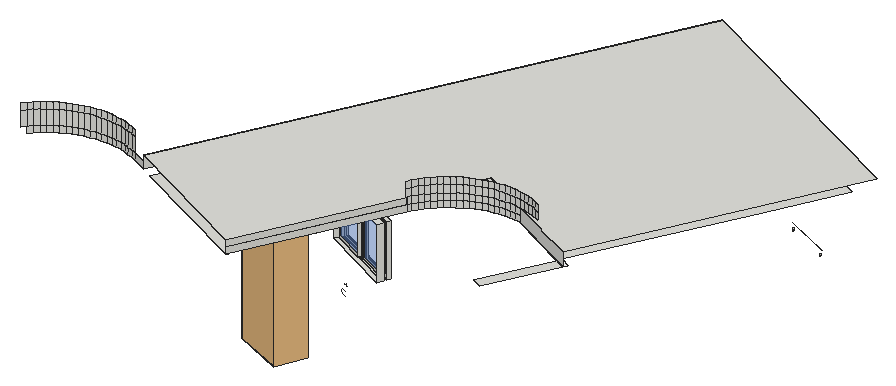
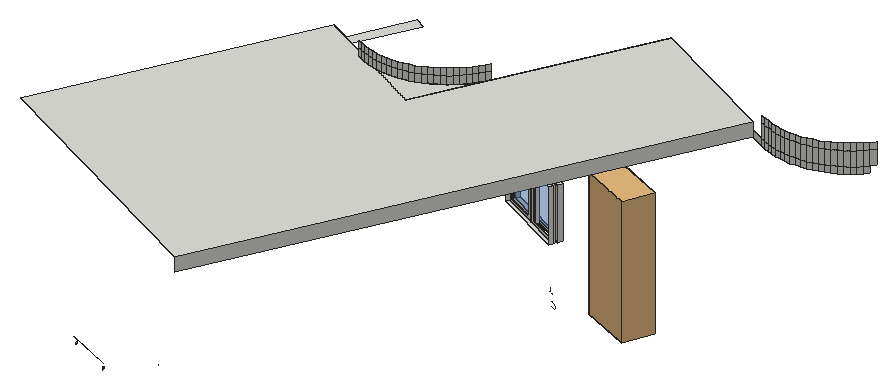
# SketchUp Ruby script. Lengths in inches.
U = 1.inch
M = Sketchup.active_model
def pt(a) = Geom::Point3d.new(a.map { |v| v * U })
def face(e, loops, mat)
  f = e.add_face(loops[0].map { |a| pt(a) })
  loops[1..].each { |l| e.add_face(l.map { |a| pt(a) }).erase! }
  f.material = f.back_material = mat if mat
  f
end
# faces: each face lists its corners as indices into pts; further lists are holes
def faces(e, pts, list, mat = nil) = list.each { |f| face(e, (f[0].is_a?(Array) ? f : [f]).map { |l| l.map { |i| pts[i] } }, mat) }
# xy, xz, yz: faces in a plane at the given z, y or x. An outline is a flat list of corners, or four numbers for a rectangle; further outlines are holes
def ring(l) = l.size == 4 ? [[l[0], l[1]], [l[2], l[1]], [l[2], l[3]], [l[0], l[3]]] : l.each_slice(2).to_a
def flat(e, list, mat, &to3) = list.each { |f| face(e, (f[0].is_a?(Array) ? f : [f]).map { |l| ring(l).map { |u, v| to3.(u, v) } }, mat) }
def xy(e, z, list, mat = nil) = flat(e, list, mat) { |x, y| [x, y, z] }
def xz(e, y, list, mat = nil) = flat(e, list, mat) { |x, z| [x, y, z] }
def yz(e, x, list, mat = nil) = flat(e, list, mat) { |y, z| [x, y, z] }
def lines(e, pts, list) = list.each { |a, b| e.add_line(pt(pts[a]), pt(pts[b])) }
# prism: a flat outline (further loops are holes) pulled along v
def prism(e, loops, v, mat = nil)
  f = face(e, loops, mat); d = Geom::Vector3d.new(v.map { |x| x * U })
  f.pushpull(f.normal.samedirection?(d) ? d.length : -d.length)
end
def box(e, o, s, mat = nil) = prism(e, [[o, [o[0] + s[0], o[1], o[2]], [o[0] + s[0], o[1] + s[1], o[2]], [o[0], o[1] + s[1], o[2]]]], [0, 0, s[2]], mat)
def at(x, y, z, deg = 0) = Geom::Transformation.translation(pt([x, y, z])) * Geom::Transformation.rotation(ORIGIN, Z_AXIS, deg.degrees)
def axes(o, x, y, z) = Geom::Transformation.new([*x, 0, *y, 0, *z, 0, *pt(o).to_a, 1])
def part(name) = M.definitions.add(name)
# library, detail: a bought-in or finely detailed component or shape, given as its bounding box
def library(name, o, s) = part(name).tap { |d| box(d.entities, o, s) }
def detail(e, o, s) = box(e.add_group.entities, o, s)
def put(e, d, t, mat = nil) = e.add_instance(d, t).tap { |i| i.material = mat if mat }
def group(e, t, mat = nil) = e.add_group.tap { |g| g.transformation = t; g.material = mat if mat }.entities
root = M.entities
M.materials.add("Glass_Safety_01").color = [204, 235, 244]
M.materials["Glass_Safety_01"].alpha = 0.1
M.materials.add("[Color_000]").color = [255, 255, 255]
M.materials.add("[Translucent Glass Blue]").color = [100, 149, 237]
M.materials["[Translucent Glass Blue]"].alpha = 0.5
c1 = library("Shower_03.skp",[-9.2,-8.46,-0.03],[13.92,58.47,24.25])
c2 = part("Janela aluminio")
xy(c2.entities,0,[[0,0,47.24,1.57],[23.62,1.57,47.24,2.76],[0,2.76,25.98,3.9375],[0,3.9375,47.24,5.91]])
xy(c2.entities,43.31,[[0,0,47.24,1.57],[23.62,1.57,47.24,2.76],[0,2.76,0,5.91,47.24,5.91,47.24,3.9375,25.98,3.9375,25.98,2.76],[25.98,2.76,47.24,3.9375]])
xz(c2.entities,1.57,[[0,0,23.62,0,23.62,41.34,21.26,41.34,21.26,1.97,1.97,1.97,1.97,41.34,23.62,41.34,23.62,43.31,0,43.31],[[23.62,0,47.24,43.31],[25.7,1.97,45.28,41.34]]])
xz(c2.entities,2.76,[[[0,0,23.62,43.31],[2.36,2.36,21.26,40.94]],[23.62,0,25.98,43.31]])
xz(c2.entities,2.76,[[2.36,2.36,21.26,40.94]],"[Translucent Glass Blue]")
xz(c2.entities,3.9375,[[25.98,0,25.98,2.36,44.88,2.36,44.88,40.94,25.98,40.94,25.98,43.31,47.24,43.31,47.24,0]])
xz(c2.entities,3.9375,[[25.98,2.36,44.88,40.94]],"[Translucent Glass Blue]")
yz(c2.entities,0,[[0,0,1.57,43.31],[2.76,0,5.91,43.31]])
yz(c2.entities,23.62,[[1.57,0,2.76,43.31]])
yz(c2.entities,25.98,[[2.76,0,3.9375,43.31]])
yz(c2.entities,47.24,[[0,0,1.57,43.31],[1.57,0,2.76,43.31],[3.9375,0,5.91,43.31]])
xy(root,354.51,[[846.73,1089.54,846.8,1089.72,825.62,1098.73],[846.8,1089.72,825.7,1098.91,825.62,1098.73]],"Glass_Safety_01")
xy(root,412.84,[[744.84,871.72,744.58,871.85,776.25,937.08,776.52,936.95],[744.57,871.86,686.94,899.84,784.83,1101.43,892.64,1049.08,877.08,1017.03,841.92,944.62,824.11,953.26,821.96,954.22,819.75,955.04,817.49,955.71,815.2,956.23,812.87,956.6,790.91,967.26,776.25,937.08,776,936.6],[831.12,910.93,845.58,940.71,841.08,942.9,826.625,913.12],[776.25,937.08,790.91,967.26,812.87,956.6,810.52,956.81,808.17,956.88,805.8125,956.79,803.47,956.54,801.15,956.14,798.86,955.59,796.61,954.9,794.41,954.05,792.27,953.07,790.2,951.94,788.21,950.6875,786.3,949.3,784.49,947.8,782.78,946.18,781.18,944.45,779.69,942.62,778.33,940.7,777.1,938.6875],[841.08,942.9,812.87,956.6,815.2,956.23,817.49,955.71,819.75,955.04,821.96,954.22,824.11,953.26,841.92,944.62]])
xy(root,412.84,[[845.58,940.71,846.42,942.43,841.92,944.62,841.08,942.9]],"[Color_000]")
xy(root,415.76,[[744.84,871.72,744.57,871.86,776,936.6,776.25,937.08,776.52,936.95]])
xy(root,418.84,[[744.57,871.86,776,936.6,776.25,937.08,790.91,967.26,812.87,956.6,845.58,940.71,900.47,1053.75,783.66,1110.47,682.44,902.02],[776.25,937.08,777.1,938.6875,778.33,940.7,779.69,942.62,781.18,944.45,782.78,946.18,784.49,947.8,786.3,949.3,788.21,950.6875,790.2,951.94,792.27,953.07,794.41,954.05,796.61,954.9,798.86,955.59,801.15,956.14,803.47,956.54,805.8125,956.79,808.17,956.88,810.52,956.81,812.87,956.6,790.91,967.26]])
p = [[845.78,1089.95,352.07],[845.88,1089.9,351.8125],[845.77,1089.65,351.8125],[845.67,1089.69,352.07],[826.59,1098.3,351.8125],[826.69,1098.26,352.07],
  [826.58,1098.01,352.07],[826.48,1098.05,351.8125],[845.75,1089.96,352.35],[845.64,1089.71,352.35],[826.73,1098.25,352.35],[826.62,1097.99,352.35],
  [845.78,1089.95,352.62],[845.67,1089.69,352.62],[826.69,1098.26,352.62],[826.58,1098.01,352.62],[826.59,1098.3,352.88],[826.48,1098.05,352.88],
  [744.84,871.72,412.84],[776.52,936.95,412.84],[776.52,936.95,415.76],[744.84,871.72,415.76],[776,936.6,412.84],[744.57,871.86,412.84],
  [744.57,871.86,415.76],[776,936.6,415.76],[634.24,898.27,415.76],[634.24,898.27,412.84],[632.64,896.54,412.84],[632.64,896.54,415.76],
  [635.95,899.89,415.76],[635.95,899.89,412.84],[637.76,901.4,415.76],[637.76,901.4,412.84],[639.67,902.78,415.76],[639.67,902.78,412.84],
  [675.58,905.36,415.76],[682.44,902.02,415.76],[682.44,902.02,412.84],[675.58,905.36,412.84],[780.62,1104.21,412.84],[682.44,902.02,418.84],
  [783.66,1110.47,418.84],[783.66,1110.47,412.84],[641.66,904.04,415.76],[641.66,904.04,412.84],[643.73,905.16,415.76],[643.73,905.16,412.84],
  [645.875,906.15,415.76],[645.875,906.15,412.84],[673.43,906.3125,412.84],[673.43,906.3125,415.76],[648.07,906.99,415.76],[648.07,906.99,412.84],
  [671.22,907.13,412.84],[671.22,907.13,415.76],[650.32,907.6875,415.76],[650.32,907.6875,412.84],[668.96,907.8,412.84],[668.96,907.8,415.76],
  [652.61,908.24,415.76],[652.61,908.24,412.84],[666.66,908.32,412.84],[666.66,908.32,415.76],[654.9375,908.63,415.76],[654.9375,908.63,412.84],
  [664.33,908.69,412.84],[664.33,908.69,415.76],[657.28,908.88,415.76],[657.28,908.88,412.84],[661.99,908.91,412.84],[661.99,908.91,415.76],
  [659.63,908.97,415.76],[659.63,908.97,412.84],[776.25,937.08,415.76],[776.25,937.08,412.84],[777.1,938.6875,412.84],[777.1,938.6875,415.76],
  [790.91,967.26,412.84],[790.91,967.26,418.84],[776.25,937.08,418.84],[778.33,940.7,412.84],[778.33,940.7,415.76],[779.69,942.62,412.84],
  [779.69,942.62,415.76],[845.58,940.71,418.84],[812.87,956.6,418.84],[812.87,956.6,415.76],[812.87,956.6,412.84],[841.08,942.9,412.84],
  [845.58,940.71,412.84],[781.18,944.45,412.84],[781.18,944.45,415.76],[782.78,946.18,412.84],[782.78,946.18,415.76],[784.49,947.8,412.84],
  [784.49,947.8,415.76],[786.3,949.3,412.84],[786.3,949.3,415.76],[788.21,950.6875,412.84],[788.21,950.6875,415.76],[790.2,951.94,412.84],
  [790.2,951.94,415.76],[792.27,953.07,412.84],[792.27,953.07,415.76],[794.41,954.05,412.84],[794.41,954.05,415.76],[824.11,953.26,415.76],
  [824.11,953.26,412.84],[821.96,954.22,412.84],[821.96,954.22,415.76],[796.61,954.9,412.84],[796.61,954.9,415.76],[819.75,955.04,412.84],
  [819.75,955.04,415.76],[798.86,955.59,412.84],[798.86,955.59,415.76],[817.49,955.71,412.84],[817.49,955.71,415.76],[801.15,956.14,412.84],
  [801.15,956.14,415.76],[815.2,956.23,412.84],[815.2,956.23,415.76],[803.47,956.54,412.84],[803.47,956.54,415.76],[805.8125,956.79,412.84],
  [805.8125,956.79,415.76],[810.52,956.81,415.76],[810.52,956.81,412.84],[808.17,956.88,412.84],[808.17,956.88,415.76],[776,936.6,418.84],
  [744.57,871.86,418.84],[631.16,894.71,415.76],[631.16,894.71,422.51],[632.64,896.54,422.51],[634.24,898.27,422.51],[635.95,899.89,422.51],
  [637.76,901.4,422.51],[639.67,902.78,422.51],[641.66,904.04,422.51],[643.73,905.16,422.51],[645.875,906.15,422.51],[673.43,906.3125,422.51],
  [675.58,905.36,422.51],[648.07,906.99,422.51],[671.22,907.13,422.51],[650.32,907.6875,422.51],[668.96,907.8,422.51],[652.61,908.24,422.51],
  [666.66,908.32,422.51],[654.9375,908.63,422.51],[664.33,908.69,422.51],[657.28,908.88,422.51],[661.99,908.91,422.51],[659.63,908.97,422.51],
  [777.1,938.6875,418.84],[778.33,940.7,418.84],[779.69,942.62,418.84],[781.18,944.45,418.84],[782.78,946.18,418.84],[784.49,947.8,418.84],
  [786.3,949.3,418.84],[788.21,950.6875,418.84],[790.2,951.94,418.84],[792.27,953.07,418.84],[794.41,954.05,418.84],[821.96,954.22,422.51],
  [824.11,953.26,422.51],[796.61,954.9,418.84],[819.75,955.04,422.51],[798.86,955.59,418.84],[817.49,955.71,422.51],[801.15,956.14,418.84],
  [815.2,956.23,422.51],[803.47,956.54,418.84],[812.87,956.6,422.51],[805.8125,956.79,418.84],[810.52,956.81,418.84],[808.17,956.88,418.84],
  [777.1,938.6875,422.51],[776,936.6,422.51],[778.33,940.7,422.51],[779.69,942.62,422.51],[781.18,944.45,422.51],[782.78,946.18,422.51],
  [784.49,947.8,422.51],[786.3,949.3,422.51],[788.21,950.6875,422.51],[790.2,951.94,422.51],[792.27,953.07,422.51],[794.41,954.05,422.51],
  [796.61,954.9,422.51],[798.86,955.59,422.51],[801.15,956.14,422.51],[803.47,956.54,422.51],[805.8125,956.79,422.51],[810.52,956.81,422.51],
  [808.17,956.88,422.51],[631.16,894.71,425.53],[632.64,896.54,425.53],[634.24,898.27,425.53],[635.95,899.89,425.53],[637.76,901.4,425.53],
  [639.67,902.78,425.53],[641.66,904.04,425.53],[643.73,905.16,425.53],[645.875,906.15,425.53],[673.43,906.3125,425.53],[675.58,905.36,425.53],
  [648.07,906.99,425.53],[671.22,907.13,425.53],[650.32,907.6875,425.53],[668.96,907.8,425.53],[652.61,908.24,425.53],[666.66,908.32,425.53],
  [654.9375,908.63,425.53],[664.33,908.69,425.53],[657.28,908.88,425.53],[661.99,908.91,425.53],[659.63,908.97,425.53],[776,936.6,425.53],
  [777.1,938.6875,425.53],[778.33,940.7,425.53],[779.69,942.62,425.53],[781.18,944.45,425.53],[782.78,946.18,425.53],[784.49,947.8,425.53],
  [786.3,949.3,425.53],[788.21,950.6875,425.53],[790.2,951.94,425.53],[792.27,953.07,425.53],[794.41,954.05,425.53],[821.96,954.22,425.53],
  [824.11,953.26,425.53],[796.61,954.9,425.53],[819.75,955.04,425.53],[798.86,955.59,425.53],[817.49,955.71,425.53],[801.15,956.14,425.53],
  [815.2,956.23,425.53],[803.47,956.54,425.53],[812.87,956.6,425.53],[805.8125,956.79,425.53],[810.52,956.81,425.53],[808.17,956.88,425.53],
  [729.23,959.8,356.46],[729.1875,959.88,356.41],[729.16,959.95,356.4],[729.34,959.68,356.5],[729.48,959.59,356.52],[729.63,959.54,356.5],
  [729.8,959.53,356.46],[729.88,959.55,356.41],[807.75,1089.6,356.52],[807.61,1089.69,356.5],[729.59,959.82,353.41],[727.82,960.68,353.41],
  [729.14,960.04,351.28],[729.59,959.82,351.28],[727.57,960.8,353.37],[727.34,960.91,353.27],[727.14,961.01,353.1],[726.99,961.08,352.88],
  [726.86,961.14,352.35],[726.89,961.13,352.07],[726.99,961.08,351.81],[727.14,961.01,351.59],[727.34,960.91,351.43],[727.57,960.8,351.32],
  [727.82,960.68,351.28],[731.11,958.44,357.01],[731.09,958.41,357.27],[731.11,958.44,357.52],[731.15,958.53,357.76],[731.22,958.67,357.96],
  [731.31,958.85,356.41],[731.22,958.67,356.57],[731.15,958.53,356.78]]
faces(root,p,[[0,1,2,3],[4,5,6,7],[8,0,3,9],[5,10,11,6],[12,8,9,13],[10,14,15,11],[14,16,17,15],[18,19,20,21],
  [22,23,24,25],[26,27,28,29],[30,31,27,26],[32,33,31,30],[34,35,33,32],[36,37,38,39],[40,38,37,41,42,43],[44,45,35,34],
  [46,47,45,44],[48,49,47,46],[36,39,50,51],[52,53,49,48],[51,50,54,55],[56,57,53,52],[55,54,58,59],[60,61,57,56],
  [59,58,62,63],[64,65,61,60],[63,62,66,67],[68,69,65,64],[67,66,70,71],[72,73,69,68],[71,70,73,72],[25,74,75,22],
  [75,76,77,74],[75,78,79,80,74],[81,82,77,76],[83,84,82,81],[85,86,87,88,89,90],[91,92,84,83],[93,94,92,91],[95,96,94,93],
  [97,98,96,95],[99,100,98,97],[101,102,100,99],[103,104,102,101],[105,106,104,103],[107,108,109,110],[111,112,106,105],[110,109,113,114],
  [115,116,112,111],[114,113,117,118],[119,120,116,115],[118,117,121,122],[123,124,120,119],[122,121,88,87],[125,126,124,123],[88,87,86,79,78],
  [88,87,127,128],[129,130,126,125],[128,127,130,129],[24,25,131,132],[29,133,134,135],[26,29,135,136],[30,26,136,137],[32,30,137,138],
  [34,32,138,139],[44,34,139,140],[46,44,140,141],[48,46,141,142],[36,51,143,144],[52,48,142,145],[51,55,146,143],[56,52,145,147],
  [55,59,148,146],[60,56,147,149],[59,63,150,148],[64,60,149,151],[63,67,152,150],[68,64,151,153],[67,71,154,152],[72,68,153,155],
  [71,72,155,154],[131,25,74,80],[74,80,156,77],[77,156,157,82],[82,157,158,84],[84,158,159,92],[92,159,160,94],[94,160,161,96],
  [96,161,162,98],[98,162,163,100],[100,163,164,102],[102,164,165,104],[104,165,166,106],[107,110,167,168],[106,166,169,112],[110,114,170,167],
  [112,169,171,116],[114,118,172,170],[116,171,173,120],[118,122,174,172],[120,173,175,124],[122,87,86,176,174],[124,175,177,126],[127,178,86,87],
  [126,177,179,130],[130,179,178,127],[180,156,80,131,181],[182,157,156,180],[183,158,157,182],[184,159,158,183],[185,160,159,184],[186,161,160,185],
  [187,162,161,186],[188,163,162,187],[189,164,163,188],[190,165,164,189],[191,166,165,190],[192,169,166,191],[193,171,169,192],[194,173,171,193],
  [195,175,173,194],[196,177,175,195],[176,86,178,197],[198,179,177,196],[197,178,179,198],[135,134,199,200],[136,135,200,201],[137,136,201,202],
  [138,137,202,203],[139,138,203,204],[140,139,204,205],[141,140,205,206],[142,141,206,207],[144,143,208,209],[145,142,207,210],[143,146,211,208],
  [147,145,210,212],[146,148,213,211],[149,147,212,214],[148,150,215,213],[151,149,214,216],[150,152,217,215],[153,151,216,218],[152,154,219,217],
  [155,153,218,220],[154,155,220,219],[180,181,221,222],[182,180,222,223],[183,182,223,224],[184,183,224,225],[185,184,225,226],[186,185,226,227],
  [187,186,227,228],[188,187,228,229],[189,188,229,230],[190,189,230,231],[191,190,231,232],[168,167,233,234],[192,191,232,235],[167,170,236,233],
  [193,192,235,237],[170,172,238,236],[194,193,237,239],[172,174,240,238],[195,194,239,241],[174,176,242,240],[196,195,241,243],[176,197,244,242],
  [198,196,243,245],[197,198,245,244]])
lines(root,p,[[246,247],[247,248],[249,246],[250,249],[251,250],[252,251],[253,252],[254,255],[256,257],[258,259],[257,260],[260,261],
  [261,262],[262,263],[264,265],[265,266],[266,267],[267,268],[268,269],[269,270],[271,272],[272,273],[273,274],[274,275],
  [276,277],[277,278],[278,271]])
put(root,c1,axes([707.07,940.76,345.46],[0.37601,0.92662,0],[0,0,1],[0.92662,-0.37601,0]))
put(root,c2,axes([762.92,944.73,376.84],[-0.68783,0.33399,0],[-0.4368,-0.89956,0],[0,0,0.55418]))
